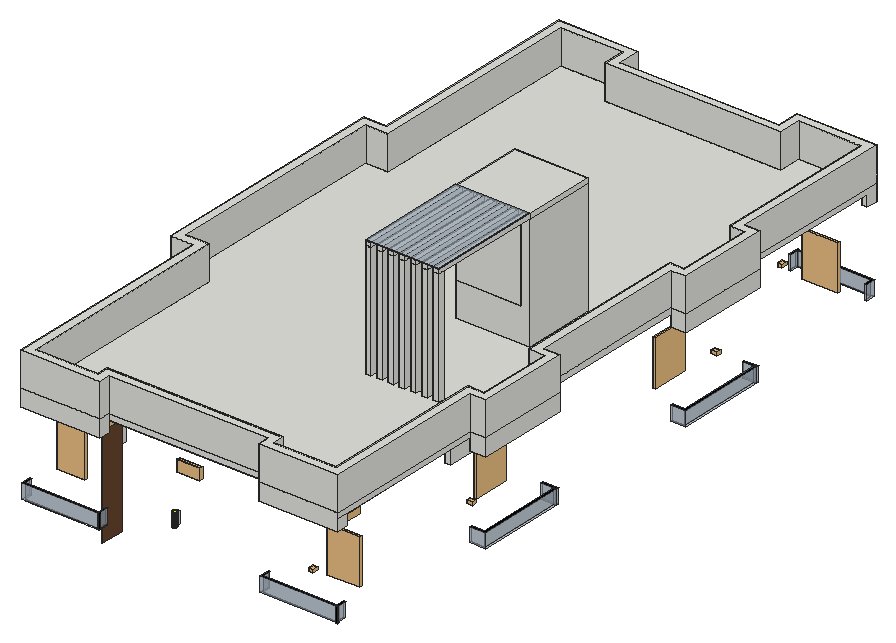
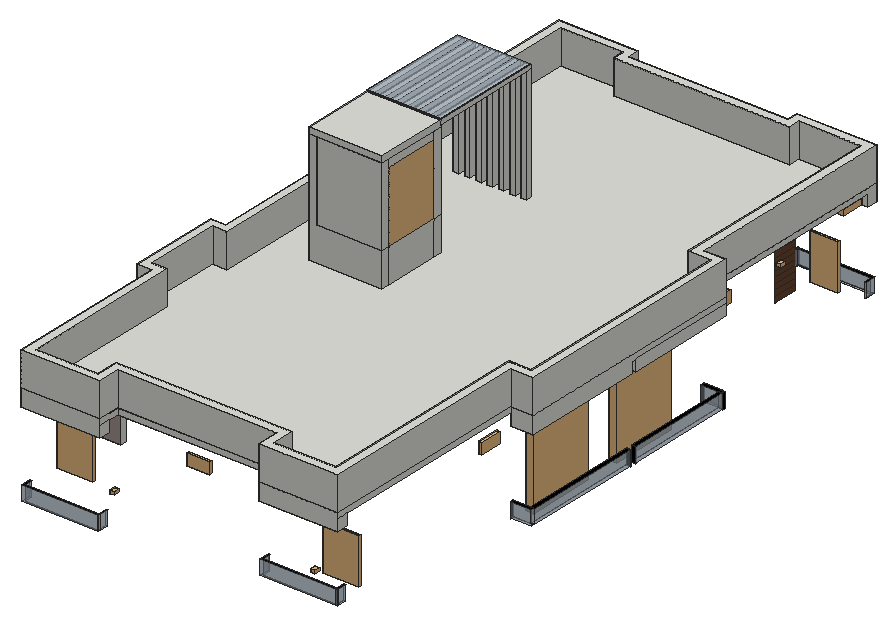
# SketchUp Ruby script. Lengths in inches.
U = 1.inch
M = Sketchup.active_model
def pt(a) = Geom::Point3d.new(a.map { |v| v * U })
def face(e, loops, mat)
  f = e.add_face(loops[0].map { |a| pt(a) })
  loops[1..].each { |l| e.add_face(l.map { |a| pt(a) }).erase! }
  f.material = f.back_material = mat if mat
  f
end
# faces: each face lists its corners as indices into pts; further lists are holes
def faces(e, pts, list, mat = nil) = list.each { |f| face(e, (f[0].is_a?(Array) ? f : [f]).map { |l| l.map { |i| pts[i] } }, mat) }
# xy, xz, yz: faces in a plane at the given z, y or x. An outline is a flat list of corners, or four numbers for a rectangle; further outlines are holes
def ring(l) = l.size == 4 ? [[l[0], l[1]], [l[2], l[1]], [l[2], l[3]], [l[0], l[3]]] : l.each_slice(2).to_a
def flat(e, list, mat, &to3) = list.each { |f| face(e, (f[0].is_a?(Array) ? f : [f]).map { |l| ring(l).map { |u, v| to3.(u, v) } }, mat) }
def xy(e, z, list, mat = nil) = flat(e, list, mat) { |x, y| [x, y, z] }
def xz(e, y, list, mat = nil) = flat(e, list, mat) { |x, z| [x, y, z] }
def yz(e, x, list, mat = nil) = flat(e, list, mat) { |y, z| [x, y, z] }
def lines(e, pts, list) = list.each { |a, b| e.add_line(pt(pts[a]), pt(pts[b])) }
# prism: a flat outline (further loops are holes) pulled along v
def prism(e, loops, v, mat = nil)
  f = face(e, loops, mat); d = Geom::Vector3d.new(v.map { |x| x * U })
  f.pushpull(f.normal.samedirection?(d) ? d.length : -d.length)
end
def box(e, o, s, mat = nil) = prism(e, [[o, [o[0] + s[0], o[1], o[2]], [o[0] + s[0], o[1] + s[1], o[2]], [o[0], o[1] + s[1], o[2]]]], [0, 0, s[2]], mat)
def at(x, y, z, deg = 0) = Geom::Transformation.translation(pt([x, y, z])) * Geom::Transformation.rotation(ORIGIN, Z_AXIS, deg.degrees)
def axes(o, x, y, z) = Geom::Transformation.new([*x, 0, *y, 0, *z, 0, *pt(o).to_a, 1])
def part(name) = M.definitions.add(name)
# library, detail: a bought-in or finely detailed component or shape, given as its bounding box
def library(name, o, s) = part(name).tap { |d| box(d.entities, o, s) }
def detail(e, o, s) = box(e.add_group.entities, o, s)
def put(e, d, t, mat = nil) = e.add_instance(d, t).tap { |i| i.material = mat if mat }
def group(e, t, mat = nil) = e.add_group.tap { |g| g.transformation = t; g.material = mat if mat }.entities
root = M.entities
M.materials.add("0-off white").color = [255, 255, 255]
M.materials.add("Glass_Basic_01").color = [161, 173, 186]
M.materials["Glass_Basic_01"].alpha = 0.59
M.materials.add("Glass_Safety_1").color = [204, 235, 244]
M.materials["Glass_Safety_1"].alpha = 0.25
M.materials.add("M09_Shadow_Night").color = [0, 0, 0]
M.materials.add("Marble_06_1K").color = [165, 150, 147]
M.materials.add("Wood_Veneer_15_1K").color = [103, 69, 45]
M.materials.add("[0056_Yellow]").color = [255, 255, 0]
c1 = library("porta correr aluminio",[0,0,0],[4.49,110.28,83.35])
c2 = part("Group\#116")
xy(c2.entities,0,[[24,0,24.75,24.75]])
xy(c2.entities,107,[[24,0,24.75,24.75]])
xz(c2.entities,0,[[24,0,24.75,107]])
xz(c2.entities,24.75,[[24,0,24.75,107]])
yz(c2.entities,24,[[0,0,24.75,6],[0,6,24.75,12],[0,12,24.75,18],[0,18,24.75,24],[0,24,24.75,30],
  [0,30,24.75,36],[0,36,24.75,42],[0,42,24.75,48],[0,48,24.75,54],[0,54,24.75,60],
  [0,60,24.75,66],[0,66,24.75,72],[0,72,24.75,78],[0,78,24.75,84],[0,84,24.75,90],
  [0,90,24.75,96],[0,96,24.75,107]],"Wood_Veneer_15_1K")
yz(c2.entities,24.75,[[0,0,24.75,107]])
c3 = part("Group\#85")
xy(c3.entities,0,[[0,0,0,11.0625,2,11.0625,2,2,80,2,80,0],[80,0,82,2],[80,2,82,11.0625]])
xy(c3.entities,16,[[0,0,80,0,80,2,2,2,2,11.0625,0,11.0625],[80,0,82,2],[80,2,82,11.0625]],"M09_Shadow_Night")
xz(c3.entities,0,[[80,0,82,16]])
xz(c3.entities,0,[[0,0,80,16]],"Glass_Basic_01")
xz(c3.entities,2,[[2,0,80,16],[80,0,82,16]])
xz(c3.entities,11.0625,[[0,0,2,16],[80,0,82,16]])
yz(c3.entities,0,[[0,0,11.0625,16]])
yz(c3.entities,2,[[2,0,11.0625,16]])
yz(c3.entities,80,[[0,0,2,16],[2,0,11.0625,16]])
yz(c3.entities,82,[[0,0,2,16],[2,0,11.0625,16]])
c4 = part("Group\#90")
xy(c4.entities,0,[[0,0,0,11.0625,2,11.0625,2,2,80,2,80,0],[80,0,82,2],[80,2,82,11.0625]])
xy(c4.entities,16,[[0,0,80,0,80,2,2,2,2,11.0625,0,11.0625],[80,0,82,2],[80,2,82,11.0625]],"M09_Shadow_Night")
xz(c4.entities,0,[[80,0,82,16]])
xz(c4.entities,0,[[0,0,80,16]],"Glass_Basic_01")
xz(c4.entities,2,[[2,0,80,16],[80,0,82,16]])
xz(c4.entities,11.0625,[[0,0,2,16],[80,0,82,16]])
yz(c4.entities,0,[[0,0,11.0625,16]])
yz(c4.entities,2,[[2,0,11.0625,16]])
yz(c4.entities,80,[[0,0,2,16],[2,0,11.0625,16]])
yz(c4.entities,82,[[0,0,2,16],[2,0,11.0625,16]])
c5 = part("Group\#87")
xy(c5.entities,0,[[0,0,0,11.0625,2,11.0625,2,2,80,2,80,0],[80,0,82,2],[80,2,82,11.0625]])
xy(c5.entities,16,[[0,0,80,0,80,2,2,2,2,11.0625,0,11.0625],[80,0,82,2],[80,2,82,11.0625]],"M09_Shadow_Night")
xz(c5.entities,0,[[0,0,80,16]],"Glass_Basic_01")
xz(c5.entities,0,[[80,0,82,16]],"M09_Shadow_Night")
xz(c5.entities,2,[[2,0,80,16],[80,0,82,16]])
xz(c5.entities,11.0625,[[0,0,2,16],[80,0,82,16]])
yz(c5.entities,0,[[0,0,11.0625,16]])
yz(c5.entities,2,[[2,0,11.0625,16]])
yz(c5.entities,80,[[0,0,2,16],[2,0,11.0625,16]])
yz(c5.entities,82,[[2,0,11.0625,16]])
yz(c5.entities,82,[[0,0,2,16]],"M09_Shadow_Night")
c6 = part("Group\#86")
xy(c6.entities,0,[[80,-8.86,82,2],[2,0,80,2]])
xy(c6.entities,16,[[80,-8.86,82,2],[2,0,80,2]],"M09_Shadow_Night")
xz(c6.entities,-8.86,[[80,0,82,16]],"M09_Shadow_Night")
xz(c6.entities,0,[[2,0,80,16]],"Glass_Basic_01")
xz(c6.entities,2,[[2,0,80,16]])
yz(c6.entities,2,[[0,0,2,16]],"M09_Shadow_Night")
yz(c6.entities,80,[[-8.86,0,0,16],[0,0,2,16]])
yz(c6.entities,82,[[-8.86,0,2,16]])
c7 = part("Group\#89")
xy(c7.entities,0,[[0,0,0,11.0625,2,11.0625,2,2,80,2,80,0],[80,0,82,2],[80,2,82,11.0625]])
xy(c7.entities,16,[[0,0,80,0,80,2,2,2,2,11.0625,0,11.0625],[80,0,82,2],[80,2,82,11.0625]],"M09_Shadow_Night")
xz(c7.entities,0,[[0,0,80,16]],"Glass_Basic_01")
xz(c7.entities,0,[[80,0,82,16]],"M09_Shadow_Night")
xz(c7.entities,2,[[2,0,80,16],[80,0,82,16]])
xz(c7.entities,11.0625,[[0,0,2,16],[80,0,82,16]])
yz(c7.entities,0,[[0,0,11.0625,16]])
yz(c7.entities,2,[[2,0,11.0625,16]])
yz(c7.entities,80,[[0,0,2,16],[2,0,11.0625,16]])
yz(c7.entities,82,[[2,0,11.0625,16]])
yz(c7.entities,82,[[0,0,2,16]],"M09_Shadow_Night")
c8 = part("Group\#88")
xy(c8.entities,0,[[2,0,80,2],[80,0,82,2],[80,2,82,11.0625]])
xy(c8.entities,16,[[2,0,80,2],[80,0,82,2],[80,2,82,11.0625]],"M09_Shadow_Night")
xz(c8.entities,0,[[2,0,80,16]],"Glass_Basic_01")
xz(c8.entities,0,[[80,0,82,16]],"M09_Shadow_Night")
xz(c8.entities,2,[[2,0,80,16],[80,0,82,16]])
xz(c8.entities,11.0625,[[80,0,82,16]],"M09_Shadow_Night")
yz(c8.entities,2,[[0,0,2,16]],"M09_Shadow_Night")
yz(c8.entities,80,[[0,0,2,16],[2,0,11.0625,16]])
yz(c8.entities,82,[[2,0,11.0625,16]])
yz(c8.entities,82,[[0,0,2,16]],"M09_Shadow_Night")
c9 = library("Slide Window 5'",[0,-2.02,0],[60,2.02,54])
c10 = library("Group\#52",[0,0,0],[4.66,6.14,3.22])
c11 = part("Wall light")
xy(c11.entities,0,[[1.3,1.93,0.875,2.1,0.51,2.38,0.23,2.74,0.06,3.17,0,3.62,0.06,4.07,0.23,4.49,0.51,4.86,0.875,5.13,1.3,5.31,1.75,5.37,2.2,5.31,2.625,5.13,2.99,4.86,3.27,4.49,3.44,4.07,3.5,3.62,3.44,3.17,3.27,2.74,2.99,2.38,2.625,2.1,2.2,1.93]],"[0056_Yellow]")
xy(c11.entities,0.74,[[1.01,0,2.57,1.93]])
xy(c11.entities,10.13,[[1.01,0,2.57,0,2.57,1.93,2.2,1.93,1.75,1.87,1.3,1.93,1.01,1.93]])
xy(c11.entities,10.875,[[1.75,1.87,2.2,1.93,1.3,1.93]])
xy(c11.entities,10.875,[[1.3,1.93,2.2,1.93,2.625,2.1,2.99,2.38,3.27,2.74,3.44,3.17,3.5,3.62,3.44,4.07,3.27,4.49,2.99,4.86,2.625,5.13,2.2,5.31,1.75,5.37,1.3,5.31,0.875,5.13,0.51,4.86,0.23,4.49,0.06,4.07,0,3.62,0.06,3.17,0.23,2.74,0.51,2.38,0.875,2.1]],"[0056_Yellow]")
xz(c11.entities,0,[[1.01,0.74,2.57,10.13]])
xz(c11.entities,1.93,[[1.3,0,2.2,0.74],[1.01,0.74,1.3,10.13],[1.3,0.74,2.2,10.875],[2.2,0.74,2.57,10.13]])
yz(c11.entities,1.01,[[0,0.74,1.93,10.13]])
yz(c11.entities,2.57,[[0,0.74,1.93,10.13]])
p = [[1.3,1.93,10.875],[0.875,2.1,10.875],[0.875,2.1,0],[1.3,1.93,0],[1.3,1.93,0.74],[1.3,1.93,10.13],
  [2.625,2.1,10.875],[2.2,1.93,10.875],[2.2,1.93,10.13],[2.2,1.93,0.74],[2.2,1.93,0],[2.625,2.1,0],
  [0.51,2.38,10.875],[0.51,2.38,0],[2.99,2.38,10.875],[2.99,2.38,0],[0.23,2.74,10.875],[0.23,2.74,0],
  [3.27,2.74,10.875],[3.27,2.74,0],[0.06,3.17,10.875],[0.06,3.17,0],[3.44,3.17,10.875],[3.44,3.17,0],
  [0,3.62,10.875],[0,3.62,0],[3.5,3.62,10.875],[3.5,3.62,0],[0.06,4.07,10.875],[0.06,4.07,0],
  [3.44,4.07,10.875],[3.44,4.07,0],[0.23,4.49,10.875],[0.23,4.49,0],[3.27,4.49,10.875],[3.27,4.49,0],
  [0.51,4.86,10.875],[0.51,4.86,0],[2.99,4.86,10.875],[2.99,4.86,0],[0.875,5.13,10.875],[0.875,5.13,0],
  [2.625,5.13,10.875],[2.625,5.13,0],[1.3,5.31,10.875],[1.3,5.31,0],[2.2,5.31,10.875],[2.2,5.31,0],
  [1.75,5.37,10.875],[1.75,5.37,0],[1.75,1.87,10.875],[1.75,1.87,10.13]]
faces(c11.entities,p,[[0,1,2,3,4,5],[6,7,8,9,10,11],[1,12,13,2],[14,6,11,15],[12,16,17,13],[18,14,15,19],[16,20,21,17],[22,18,19,23],
  [20,24,25,21],[26,22,23,27],[24,28,29,25],[30,26,27,31],[28,32,33,29],[34,30,31,35],[32,36,37,33],[38,34,35,39],
  [36,40,41,37],[42,38,39,43],[40,44,45,41],[46,42,43,47],[44,48,49,45],[48,46,47,49],[50,0,5,51],[7,50,51,8]])
c12 = part("Group\#305")
xy(c12.entities,0.81,[[0.28,-0.04,1.69,0]],"0-off white")
xz(c12.entities,-0.04,[[0.28,0.81,1.69,0.81,0.98,1.5]],"0-off white")
xz(c12.entities,0,[[[0.98,0,1.24,0.03,1.48,0.13,1.68,0.29,1.84,0.49,1.93,0.73,1.97,0.98,1.93,1.24,1.84,1.48,1.68,1.68,1.48,1.84,1.24,1.93,0.98,1.97,0.73,1.93,0.49,1.84,0.29,1.68,0.13,1.48,0.03,1.24,0,0.98,0.03,0.73,0.13,0.49,0.29,0.29,0.49,0.13,0.73,0.03],[0.28,0.81,0.98,1.5,1.69,0.81]]],"0-off white")
xz(c12.entities,0.63,[[0.98,0,0.73,0.03,0.49,0.13,0.29,0.29,0.13,0.49,0.03,0.73,0,0.98,0.03,1.24,0.13,1.48,0.29,1.68,0.49,1.84,0.73,1.93,0.98,1.97,1.24,1.93,1.48,1.84,1.68,1.68,1.84,1.48,1.93,1.24,1.97,0.98,1.93,0.73,1.84,0.49,1.68,0.29,1.48,0.13,1.24,0.03]],"0-off white")
p = [[0.49,0.63,0.13],[0.73,0.63,0.03],[0.73,0,0.03],[0.49,0,0.13],[0.98,0.63,0],[0.98,0,0],
  [1.24,0.63,0.03],[1.24,0,0.03],[1.48,0.63,0.13],[1.48,0,0.13],[0.29,0.63,0.29],[0.29,0,0.29],
  [1.68,0.63,0.29],[1.68,0,0.29],[0.13,0.63,0.49],[0.13,0,0.49],[1.84,0.63,0.49],[1.84,0,0.49],
  [0.03,0.63,0.73],[0.03,0,0.73],[1.93,0.63,0.73],[1.93,0,0.73],[0,0.63,0.98],[0,0,0.98],
  [1.97,0.63,0.98],[1.97,0,0.98],[0.98,0,1.5],[0.28,0,0.81],[0.28,-0.04,0.81],[0.98,-0.04,1.5],
  [1.69,0,0.81],[1.69,-0.04,0.81],[0.03,0.63,1.24],[0.03,0,1.24],[1.93,0.63,1.24],[1.93,0,1.24],
  [0.13,0.63,1.48],[0.13,0,1.48],[1.84,0.63,1.48],[1.84,0,1.48],[0.29,0.63,1.68],[0.29,0,1.68],
  [1.68,0.63,1.68],[1.68,0,1.68],[0.49,0.63,1.84],[0.49,0,1.84],[1.48,0.63,1.84],[1.48,0,1.84],
  [0.73,0.63,1.93],[0.73,0,1.93],[1.24,0.63,1.93],[1.24,0,1.93],[0.98,0.63,1.97],[0.98,0,1.97]]
faces(c12.entities,p,[[0,1,2,3],[1,4,5,2],[4,6,7,5],[6,8,9,7],[10,0,3,11],[8,12,13,9],[14,10,11,15],[12,16,17,13],
  [18,14,15,19],[16,20,21,17],[22,18,19,23],[20,24,25,21],[26,27,28,29],[30,26,29,31],[32,22,23,33],[24,34,35,25],
  [36,32,33,37],[34,38,39,35],[40,36,37,41],[38,42,43,39],[44,40,41,45],[42,46,47,43],[48,44,45,49],[46,50,51,47],
  [52,48,49,53],[50,52,53,51]],"0-off white")
c13 = part("Group\#370")
box(c13.entities,[0,0,-0.39],[5.12,10.31,0.39])
g1 = group(c13.entities,at(1.59,1.64,0.22))
put(g1,c12,axes([0,4.49,0],[1,0,0],[0,0,-0.35294],[0,1,0]))
put(g1,c12,axes([0,2,0],[1,0,0],[0,0,-0.35294],[0,-1,0]))
c14 = library("Group\#46",[0,-0.05,0],[30,2.55,24])
c15 = library("Group\#115",[0,0,0],[72,16,6.2])
c16 = part("Group\#103")
box(c16.entities,[0,-120,0],[6,120,6])
c17 = part("Group\#107")
box(c17.entities,[0,0,-168.1],[6,6,168.1])
c18 = library("Metal grille gate",[0,0,0],[35.98,1.97,83.98])
box(root,[119.8,217.34,455.9375],[6,30,36])
box(root,[332.2,217.34,456],[6,30,36])
box(root,[181.8,337.55,456],[6,48.35,36])
box(root,[73.8,709.34,456],[30,6,36])
box(root,[332.19,541.34,456],[6.01,30,36])
box(root,[119.8,541.34,456],[6,30,36])
box(root,[218.2,631.34,456],[6,30,36])
box(root,[181.8,391.55,456],[6,48,36])
box(root,[218.2,127.34,456],[6,30,36])
box(root,[218.2,583.34,456],[6,42,36])
box(root,[218.2,163.34,456],[6,42,36])
box(root,[163.8,583.34,456],[6,42,36])
box(root,[163.8,163.34,456],[6,38.53,36])
box(root,[233.2,364.34,609.1],[9,60,9])
xy(root,456,[[284.2,73.34,314.2,79.34],[76.2,75.06,103.8,79.34],[37.8,295.34,43.8,367.34],[37.8,404.89,43.8,476.03],[284.2,709.34,314.2,715.34]])
xy(root,492,[[284.2,73.34,314.2,79.34],[76.2,75.06,103.8,79.34],[37.8,295.34,43.8,367.34],[37.8,404.89,43.8,476.03],[284.2,709.34,314.2,715.34]])
xz(root,73.34,[[284.2,456,314.2,492]],"Marble_06_1K")
xz(root,75.06,[[76.2,456,103.8,492]],"Marble_06_1K")
xz(root,79.34,[[76.2,456,103.8,492],[284.2,456,314.2,492]])
xz(root,295.34,[[37.8,456,43.8,492]])
xz(root,367.34,[[37.8,456,43.8,492]])
xz(root,404.89,[[37.8,456,43.8,492]])
xz(root,476.03,[[37.8,456,43.8,492]])
xz(root,709.34,[[284.2,456,314.2,492]])
xz(root,715.34,[[284.2,456,314.2,492]],"Marble_06_1K")
yz(root,37.8,[[295.34,456,367.34,492],[404.89,456,476.03,492]],"Marble_06_1K")
yz(root,43.8,[[295.34,456,367.34,492],[404.89,456,476.03,492]])
yz(root,76.2,[[75.06,456,79.34,492]])
yz(root,103.8,[[75.06,456,79.34,492]])
yz(root,284.2,[[73.34,456,79.34,492],[709.34,456,715.34,492]])
yz(root,314.2,[[73.34,456,79.34,492],[709.34,456,715.34,492]])
p = [[181.8,49.34,468],[181.8,49.34,480],[206.2,49.34,480],[206.2,49.34,468],[278.2,739.27,498],[278.2,727.34,498],
  [109.91,727.34,498],[109.91,739.27,498],[108.8,38.27,392],[28.8,38.27,392],[106.8,40.27,392],[106.8,49.34,392],
  [108.8,49.34,392],[28.8,40.27,392],[242.2,364.34,582.1],[233.2,364.34,582.1],[242.2,424.34,582.1],[233.2,424.34,582.1]]
lines(root,p,[[0,1],[1,2],[2,3],[3,0],[4,5],[5,6],[6,7],[8,9],[10,11],[8,12],[13,10],[14,15],
  [16,17]])
put(root,c1,axes([45.93,404.95,372.65],[-1.89519,0,0],[0,0.65291,0],[0,0,1]))
put(root,c1,axes([45.93,295.34,372.65],[-1.89519,0,0],[0,0.65291,0],[0,0,1]))
put(root,c2,axes([79.05,49.34,373],[1,0,0],[0,1.02586,0],[0,0,1.00467]),"Wood_Veneer_15_1K")
put(root,c3,axes([377.67,479.34,390],[0,1.18,0],[-1.39867,0,0],[0,0,1]),"Glass_Basic_01")
put(root,c4,at(361.2,750.33,390,180),"Glass_Basic_01")
put(root,c5,at(26.8,38.27,392),"Glass_Basic_01")
put(root,c6,axes([6.91,388.28,392],[0,1.63485,0],[-2.08447,0,0],[0,0,1]),"Glass_Basic_01")
put(root,c3,axes([379.2,212.34,392],[0,1.18,0],[-1.537,0,0],[0,0,1]),"Glass_Basic_01")
put(root,c7,at(279.2,38.27,392),"Glass_Basic_01")
put(root,c8,axes([2.74,388.52,392],[0,-1.49,0],[2.08447,0,0],[0,0,1]),"Glass_Basic_01")
put(root,c9,axes([337.02,292.34,407.33],[0,-0.65004,0],[1.4091,0,0],[0,0,0.88889]))
put(root,c9,axes([336.93,529.39,407.94],[0,-0.65094,0],[1.4091,0,0],[0,0,0.88889]))
put(root,c9,axes([64.2,75.12,408],[-0.49488,0,0],[0,-1.4091,0],[0,0,0.89778]))
put(root,c9,axes([33.8,713.23,408],[0.63333,0,0],[0,1.4091,0],[0,0,0.88889]))
put(root,c9,axes([355.2,75.12,408],[-0.58385,0,0],[0,-1.4091,0],[0,0,0.88889]))
put(root,c9,axes([316.2,713.15,408],[0.63333,0,0],[0,1.4091,0],[0,0,0.88889]))
put(root,c4,at(108.8,750.33,408,180),"Glass_Basic_01")
put(root,c10,at(101.8,75.06,408.64,180))
put(root,c10,at(336.48,245.16,408.75,-90))
put(root,c10,at(336.48,569.34,408.75,-90))
put(root,c10,at(287.63,713.62,408.75))
put(root,c10,at(75.08,713.8,408.89))
put(root,c10,at(312.2,73.34,410.0625,180))
put(root,c11,axes([186.48,49.34,419],[-1.35,0,0],[0,-1.35,0],[0,0,1.35]))
put(root,c13,axes([236.2,421.93,422.05],[0,-0.53664,0],[0,0,1],[-1.59369,0,0]))
put(root,c14,axes([26.6,253.34,468],[0,-0.8,0],[1.27878,0,0],[0,0,0.5]))
put(root,c14,axes([206.2,725.55,468],[-0.81341,0,0],[0,-1.27878,0],[0,0,0.5]))
put(root,c14,axes([26.6,559.34,468],[0,-0.8,0],[1.27878,0,0],[0,0,0.5]))
put(root,c14,axes([181.8,50.02,468],[0.81333,0,0],[0,1.27878,0],[0,0,0.5]))
put(root,c15,axes([5.8,385.9,485.5],[0,-1.5912,0],[2,0,0],[0,0,-1]))
put(root,c15,axes([285.28,41.34,485.86],[1,0,0],[0,2,0],[0,0,-1]))
put(root,c15,axes([31.8,41.34,486],[1,0,0],[0,2,0],[0,0,-1]))
g2 = group(root,at(25.8,49.34,516.53))
xy(g2,-36.67,[[252.4,-12,252.4,0,259.49,0,259.49,-8,330.4,-8,330.4,0,336.4,0,336.4,-12]])
xy(g2,-36.53,[[0,-12,0,-0.08,6,-0.08,6,-8,78,-8,78,0,84,0,84,-12],[336.4,163,336.4,169,349.41,169,349.41,255,336.4,255,336.4,261,353.41,261,353.41,163],[-24,217,-24,336.57,-20,336.57,-20,222,0,222,0,217],[-24,342.21,-24,473,0,473,0,468,-20,468,-20,342.21],[336.4,430,336.4,435,347.875,435,347.875,523,335.62,523,335.62,528,351.875,528,351.875,430],
  [0,689.93,0,701.93,84,701.93,84,689.93,78,689.93,78,697.93,6,697.93,6,689.93],[252.4,689.93,252.4,701.93,336.4,701.93,336.4,689.93,330.4,689.93,330.4,697.93,258.4,697.93,258.4,689.93]])
xy(g2,-24.53,[[[6,-8,6,-0.08,0,-0.08,0,222,-20,222,-20,336.57,-24,336.57,-24,342.21,-20,342.21,-20,468,0,468,0,689.93,6,689.93,6,697.93,78,697.93,78,689.93,84,689.93,84,678,252.4,678,252.4,689.93,258.4,689.93,258.4,697.93,330.4,697.93,330.4,689.93,336.4,689.93,336.4,528,335.62,528,335.62,523,347.875,523,347.875,435,336.4,435,336.4,255,349.41,255,349.41,169,336.4,169,336.4,0,330.4,0,330.4,-8,259.49,-8,259.49,0,78,0,78,-8],[216.4,315,276.4,375]],[-24,217,0,217,0,222,-20,222,-20,336.57,-24,336.57]])
xy(g2,-18.53,[[[9,-3,75,-3,75,9,261.4,9,261.4,-3,327.4,-3,327.4,172,344.41,172,344.41,252,327.4,252,327.4,439,342.875,439,342.875,519,327.4,519,327.4,692.93,261.4,692.93,261.4,669,75,669,75,692.93,9,692.93,9,464,-15,464,-15,226,9,226],[207.4,306,285.4,384]]])
xy(g2,17.58,[[207.4,306,276.4,315],[207.4,315,216.4,375],[267.4,315,276.4,375],[207.4,375,276.4,384]])
xy(g2,101.58,[[207.4,306,276.4,306,276.4,384,207.4,384,207.4,375,267.4,375,267.4,315,207.4,315],[276.4,306,285.4,375],[276.4,375,285.4,384]])
xz(g2,-12,[[252.4,-36.67,336.4,-18.53],[0,-36.53,84,-18.53]])
xz(g2,-8,[[259.49,-36.67,330.4,-24.53],[6,-36.53,78,-24.53]])
xz(g2,-0.08,[[0,-36.53,6,-24.53]])
xz(g2,0,[[252.4,-36.67,259.49,-24.53],[330.4,-36.67,336.4,-24.53],[78,-36.53,84,-24.53],[84,-24.53,252.4,-18.53]])
xz(g2,163,[[336.4,-36.53,353.41,-18.53]])
xz(g2,169,[[336.4,-36.53,349.41,-24.53]])
xz(g2,217,[[-24,-36.53,0,-24.53],[-24,-24.53,0,-18.53]])
xz(g2,222,[[-20,-36.53,0,-24.53]])
xz(g2,255,[[336.4,-36.53,349.41,-24.53]])
xz(g2,261,[[336.4,-36.53,353.41,-18.53]])
xz(g2,306,[[207.4,-18.53,285.4,-18.53,285.4,101.58,276.4,101.58,276.4,17.58,207.4,17.58],[207.4,17.58,276.4,101.58]])
xz(g2,315,[[216.4,-24.53,276.4,17.58],[207.4,17.58,267.4,101.58]])
xz(g2,336.57,[[-24,-36.53,-20,-24.53]])
xz(g2,342.21,[[-24,-36.53,-20,-24.53]])
xz(g2,375,[[216.4,-24.53,276.4,17.58],[207.4,17.58,267.4,101.58]])
xz(g2,384,[[207.4,-18.53,207.4,17.58,276.4,17.58,276.4,101.58,285.4,101.58,285.4,-18.53],[207.4,17.58,276.4,101.58]])
xz(g2,430,[[336.4,-36.53,351.875,-18.53]])
xz(g2,435,[[336.4,-36.53,347.875,-24.53]])
xz(g2,468,[[-20,-36.53,0,-24.53]])
xz(g2,473,[[-24,-36.53,0,-18.53]])
xz(g2,523,[[335.62,-36.53,347.875,-24.53]])
xz(g2,528,[[335.62,-36.53,351.875,-24.53],[336.4,-24.53,351.875,-18.53]])
xz(g2,678,[[84,-24.53,252.4,-18.53]])
xz(g2,689.93,[[0,-36.53,6,-24.53],[78,-36.53,84,-24.53],[252.4,-36.53,258.4,-24.53],[330.4,-36.53,336.4,-24.53]])
xz(g2,697.93,[[6,-36.53,78,-24.53],[258.4,-36.53,330.4,-24.53]])
xz(g2,701.93,[[0,-36.53,84,-18.53],[252.4,-36.53,336.4,-18.53]])
yz(g2,-24,[[217,-36.53,336.57,-24.53],[342.21,-36.53,342.21,-24.53,217,-24.53,217,-18.53,473,-18.53,473,-36.53]])
yz(g2,-20,[[222,-36.53,336.57,-24.53],[342.21,-36.53,468,-24.53]])
yz(g2,0,[[-12,-36.53,-12,-18.53,217,-18.53,217,-24.53,-0.08,-24.53,-0.08,-36.53],[217,-36.53,222,-24.53],[468,-36.53,473,-24.53],[689.93,-36.53,701.93,-24.53],[473,-24.53,701.93,-18.53]])
yz(g2,6,[[-8,-36.53,-0.08,-24.53],[689.93,-36.53,697.93,-24.53]])
yz(g2,78,[[-8,-36.53,0,-24.53],[689.93,-36.53,697.93,-24.53]])
yz(g2,84,[[-12,-36.53,0,-18.53],[689.93,-36.53,701.93,-36.53,701.93,-18.53,678,-18.53,678,-24.53,689.93,-24.53]])
yz(g2,207.4,[[306,-18.53,315,17.58],[315,-18.53,375,17.58],[375,-18.53,384,17.58],[306,17.58,315,101.58],[375,17.58,384,101.58]])
yz(g2,216.4,[[315,-24.53,375,17.58]])
yz(g2,252.4,[[-12,-36.67,0,-18.53],[689.93,-36.53,701.93,-24.53],[678,-24.53,701.93,-18.53]])
yz(g2,258.4,[[689.93,-36.53,697.93,-24.53]])
yz(g2,259.49,[[-8,-36.67,0,-24.53]])
yz(g2,267.4,[[315,17.58,375,101.58]])
yz(g2,276.4,[[315,-24.53,375,17.58],[306,17.58,315,101.58],[315,17.58,375,101.58],[375,17.58,384,101.58]])
yz(g2,285.4,[[306,-18.53,384,101.58]])
yz(g2,330.4,[[-8,-36.67,0,-24.53],[689.93,-36.53,697.93,-24.53]])
yz(g2,335.62,[[523,-36.53,528,-24.53]])
yz(g2,336.4,[[-12,-36.67,0,-24.53],[163,-36.53,169,-24.53],[255,-36.53,261,-24.53],[430,-36.53,435,-24.53],[689.93,-36.53,701.93,-36.53,701.93,-18.53,528,-18.53,528,-24.53,689.93,-24.53],
  [-12,-24.53,163,-18.53],[261,-24.53,430,-18.53]])
yz(g2,347.875,[[435,-36.53,523,-24.53]])
yz(g2,349.41,[[169,-36.53,255,-24.53]])
yz(g2,351.875,[[430,-36.53,528,-18.53]])
yz(g2,353.41,[[163,-36.53,261,-18.53]])
g3 = group(g2,at(-24,-12,-18.53))
prism(g3,[[[108,0,0],[24,0,0],[24,229,0],[0,229,0],[0,485,0],[24,485,0],[24,713.93,0],[108,713.93,0],[108,690,0],[276.4,690,0],[276.4,713.93,0],[360.4,713.93,0],[360.4,540,0],[375.875,540,0],[375.875,442,0],[360.4,442,0],[360.4,273,0],[377.41,273,0],[377.41,175,0],[360.4,175,0],[360.4,0,0],[276.4,0,0],[276.4,12,0],[108,12,0]],[[9,476,0],[9,238,0],[33,238,0],[33,9,0],[99,9,0],[99,21,0],[285.4,21,0],[285.4,9,0],[351.4,9,0],[351.4,184,0],[368.41,184,0],[368.41,264,0],[351.4,264,0],[351.4,451,0],[366.875,451,0],[366.875,531,0],[351.4,531,0],[351.4,704.93,0],[285.4,704.93,0],[285.4,681,0],[99,681,0],[99,704.93,0],[33,704.93,0],[33,476,0]]],[0,0,36])
put(root,c15,axes([5.8,385.9,486.2],[0,-1.5912,0],[2,0,0],[0,0,-1]))
put(root,c15,axes([5.8,506.12,486.2],[0,-1.5912,0],[2,0,0],[0,0,-1]))
g4 = group(root,at(233.2,235.34,498))
put(g4,c16,axes([24,120,121.76],[1,0,0],[0,1,0],[0,0,0.7243]))
put(g4,c16,axes([36,120,121.76],[1,0,0],[0,1,0],[0,0,0.7243]))
put(g4,c16,axes([12,120,121.76],[1,0,0],[0,1,0],[0,0,0.7243]))
put(g4,c16,axes([60,120,121.76],[1,0,0],[0,1,0],[0,0,0.7243]))
put(g4,c17,axes([24,0,121.76],[1,0,0],[0,1,0],[0,0,0.7243]))
put(g4,c17,axes([36,0,121.76],[1,0,0],[0,1,0],[0,0,0.7243]))
put(g4,c17,axes([0,0,121.76],[1,0,0],[0,1,0],[0,0,0.7243]))
put(g4,c17,axes([48,0,121.76],[1,0,0],[0,1,0],[0,0,0.7243]))
put(g4,c16,axes([72,120,121.76],[1,0,0],[0,1,0],[0,0,0.7243]))
put(g4,c16,axes([48,120,121.76],[1,0,0],[0,1,0],[0,0,0.7243]))
put(g4,c17,axes([12,0,121.76],[1,0,0],[0,1,0],[0,0,0.7243]))
put(g4,c16,axes([0,120,121.76],[1,0,0],[0,1,0],[0,0,0.7243]))
put(g4,c17,axes([60,0,121.76],[1,0,0],[0,1,0],[0,0,0.7243]))
put(g4,c17,axes([72,0,121.76],[1,0,0],[0,1,0],[0,0,0.7243]))
put(root,c18,axes([233.2,424.34,534.1],[0,-1.6674,0],[2,0,0],[0,0,0.89311]))
g5 = group(root,at(233.2,355.34,618.1))
box(g5,[0,0,0],[78,78,6])
g6 = group(root,at(233.2,235.34,624.1),"Glass_Safety_1")
xy(g6,0,[[0,0,78,120]])
xy(g6,1,[[0,0,78,120]],"Glass_Basic_01")
xz(g6,0,[[0,0,78,1]])
xz(g6,120,[[0,0,78,1]])
yz(g6,0,[[0,0,120,1]])
yz(g6,78,[[0,0,120,1]])
